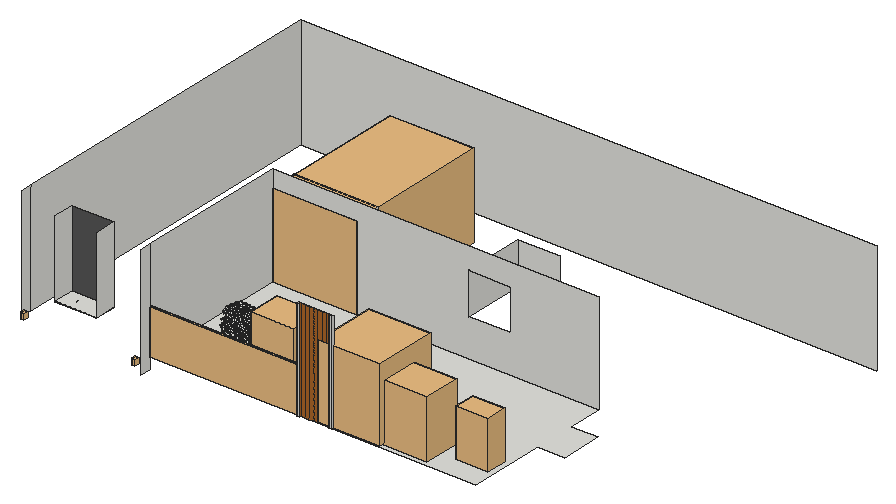
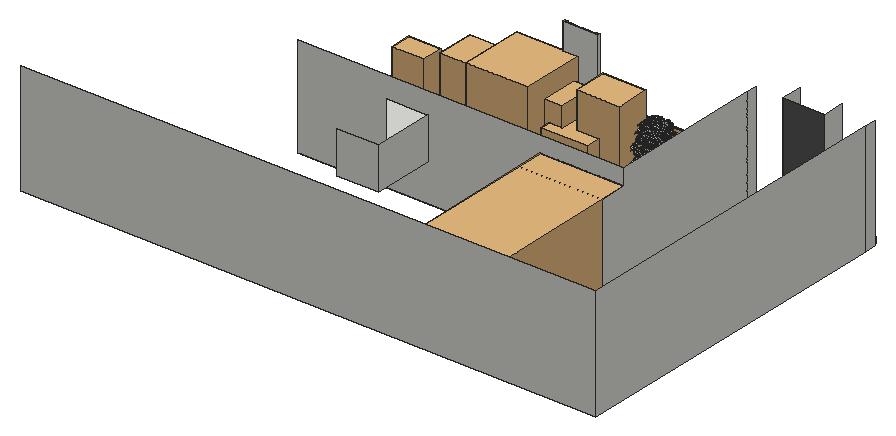
# SketchUp Ruby script. Lengths in inches.
U = 1.inch
M = Sketchup.active_model
def pt(a) = Geom::Point3d.new(a.map { |v| v * U })
def face(e, loops, mat)
  f = e.add_face(loops[0].map { |a| pt(a) })
  loops[1..].each { |l| e.add_face(l.map { |a| pt(a) }).erase! }
  f.material = f.back_material = mat if mat
  f
end
# faces: each face lists its corners as indices into pts; further lists are holes
def faces(e, pts, list, mat = nil) = list.each { |f| face(e, (f[0].is_a?(Array) ? f : [f]).map { |l| l.map { |i| pts[i] } }, mat) }
# xy, xz, yz: faces in a plane at the given z, y or x. An outline is a flat list of corners, or four numbers for a rectangle; further outlines are holes
def ring(l) = l.size == 4 ? [[l[0], l[1]], [l[2], l[1]], [l[2], l[3]], [l[0], l[3]]] : l.each_slice(2).to_a
def flat(e, list, mat, &to3) = list.each { |f| face(e, (f[0].is_a?(Array) ? f : [f]).map { |l| ring(l).map { |u, v| to3.(u, v) } }, mat) }
def xy(e, z, list, mat = nil) = flat(e, list, mat) { |x, y| [x, y, z] }
def xz(e, y, list, mat = nil) = flat(e, list, mat) { |x, z| [x, y, z] }
def yz(e, x, list, mat = nil) = flat(e, list, mat) { |y, z| [x, y, z] }
def lines(e, pts, list) = list.each { |a, b| e.add_line(pt(pts[a]), pt(pts[b])) }
# prism: a flat outline (further loops are holes) pulled along v
def prism(e, loops, v, mat = nil)
  f = face(e, loops, mat); d = Geom::Vector3d.new(v.map { |x| x * U })
  f.pushpull(f.normal.samedirection?(d) ? d.length : -d.length)
end
def box(e, o, s, mat = nil) = prism(e, [[o, [o[0] + s[0], o[1], o[2]], [o[0] + s[0], o[1] + s[1], o[2]], [o[0], o[1] + s[1], o[2]]]], [0, 0, s[2]], mat)
def at(x, y, z, deg = 0) = Geom::Transformation.translation(pt([x, y, z])) * Geom::Transformation.rotation(ORIGIN, Z_AXIS, deg.degrees)
def axes(o, x, y, z) = Geom::Transformation.new([*x, 0, *y, 0, *z, 0, *pt(o).to_a, 1])
def part(name) = M.definitions.add(name)
# library, detail: a bought-in or finely detailed component or shape, given as its bounding box
def library(name, o, s) = part(name).tap { |d| box(d.entities, o, s) }
def detail(e, o, s) = box(e.add_group.entities, o, s)
def put(e, d, t, mat = nil) = e.add_instance(d, t).tap { |i| i.material = mat if mat }
def group(e, t, mat = nil) = e.add_group.tap { |g| g.transformation = t; g.material = mat if mat }.entities
root = M.entities
M.materials.add("[Color M06]").color = [86, 86, 86]
M.materials.add("[Wood Bamboo]").color = [173, 103, 41]
c1 = library("Lamp Wall Outdoor 94-02",[-1.89,-4.65,-3.17],[3.78,4.65,6.35])
c2 = library("Omni Light",[-12,-12,-12],[24,24,24])
c3 = library("Group\#14",[0,0,0],[39.5,117.4375,51.17])
c4 = library("Glass Railings(black Handrails)",[-57.04,-132.55,0],[169.29,2.52,28.17])
c5 = library("Hanging Plant\#2",[-3.24,-1.74,-0.87],[34.15,22.4,50.98])
c6 = library("Yukka Plant GHD",[0,0,0],[46.13,35.26,75.51])
c7 = library("Philodendron Plant GHD",[-18.43,-10.97,-1.09],[51.75,39.48,62.43])
c8 = library("Plant Banana",[3.49,5.74,0],[38.27,39.55,56.51])
c9 = library("Potted indoor plant",[-35.72,-28.42,0],[66.31,67.39,78.4375])
c10 = part("leaflet")
p = [[2.87,10.24,0.32],[0.33,13.79,0],[-2.24,10.39,0.32],[-2.2,6.92,0.33],[0.45,0.11,0.33],[2.91,6.86,0.33]]
faces(c10.entities,p,[[0,1,2],[0,2,3,4,5]])
c11 = part("leaf group")
put(c11.entities,c10,axes([4.25,4.04,0.04],[0.8,0,0],[0,0.8,0],[0,0,0.8]))
put(c11.entities,c10,axes([4.5,3.78,0.04],[0.4,0.69282,-0.00011],[-0.69282,0.4,-0.00008],[-0.00001,0.00014,0.8]))
put(c11.entities,c10,axes([4.92,3.9375,0.04],[-0.56569,0.56569,-0.00025],[-0.56569,-0.56569,0.00001],[-0.00017,0.00019,0.8]))
put(c11.entities,c10,axes([4.87,4.38,0.04],[-0.69282,-0.4,-0.0002],[0.4,-0.69282,0.00017],[-0.00026,0.00005,0.8]))
put(c11.entities,c10,axes([4.42,4.45,0.04],[0.20706,-0.77274,-0.00003],[0.77274,0.20706,0.00016],[-0.00015,-0.00007,0.8]))
c12 = part("branch with leaves\#1")
put(c12.entities,c11,axes([2.86,31.23,35.15],[-0.02765,-0.79009,-0.61237],[0.48114,-0.54749,0.68465],[-0.8762,-0.27571,0.39528]))
put(c12.entities,c11,axes([12.72,29.5,24.05],[-0.41566,0.90952,0],[-0.44736,-0.20444,-0.87067],[-0.7919,-0.3619,0.49186]))
put(c12.entities,c11,axes([15.91,15.09,15.29],[-0.51919,0.82474,-0.22414],[0.78767,0.35997,-0.5],[-0.33169,-0.43615,-0.83652]))
put(c12.entities,c11,axes([23.4,16.37,17.31],[0.5,0.75,-0.43301],[0,0.5,0.86603],[0.86603,-0.43301,0.25]))
put(c12.entities,c11,axes([11.3125,8.27,23.62],[1.15,0,0],[0,0.575,0.99593],[0,-0.86603,0.5]))
c13 = part("leaflet\#1")
p = [[0.33,13.79,0],[2.87,10.24,0.32],[-2.24,10.39,0.32],[2.91,6.86,0.33],[0.45,0.11,0.33],[-2.2,6.92,0.33]]
faces(c13.entities,p,[[0,1,2],[2,1,3,4,5]])
c14 = part("leaf group\#1")
put(c14.entities,c13,axes([1.8,0.82,0.04],[-0.56569,0.56569,-0.00025],[-0.33941,-0.33941,0.00001],[-0.00017,0.00019,0.8]))
c15 = part("flower")
put(c15.entities,c14,axes([3.87,3.58,0.87],[0.08758,0.98061,-0.17532],[0.93721,-0.14075,-0.31909],[-0.33758,-0.13637,-0.93137]))
put(c15.entities,c14,axes([3.58,5.87,0.87],[0.98061,-0.08758,-0.17532],[-0.14075,-0.93721,-0.31909],[-0.13637,0.33758,-0.93137]))
put(c15.entities,c14,axes([5.87,6.16,0.87],[-0.08758,-0.98061,-0.17532],[-0.93721,0.14075,-0.31909],[0.33758,0.13637,-0.93137]))
put(c15.entities,c14,axes([6.16,3.87,0.87],[-0.98061,0.08758,-0.17532],[0.14075,0.93721,-0.31909],[0.13637,-0.33758,-0.93137]))
put(c15.entities,c14,axes([4.97,4.02,1.64],[-0.54077,0.62855,-0.55902],[0.78035,0.12673,-0.61237],[-0.31406,-0.76738,-0.55902]))
put(c15.entities,c14,axes([4.08,5.2,1.64],[0.81472,0.15405,-0.55902],[-0.28042,-0.73917,-0.61237],[-0.50754,0.65567,-0.55902]))
put(c15.entities,c14,axes([5.55,5.38,1.64],[-0.27395,-0.78259,-0.55902],[-0.49993,0.61243,-0.61237],[0.8216,0.11171,-0.55902]))
c16 = part("branch")
p = [[0.27,0.14,21.6],[1.15,1.36,21.6],[2.31,4.21,0],[0.54,1.79,0],[1.05,2.55,32.4],[1.34,2.95,32.4]]
faces(c16.entities,p,[[0,1,2,3],[4,5,1,0]])
c17 = part("branch with leaves")
put(c17.entities,c11,axes([29.28,4.46,29.75],[0.70711,0.61237,-0.35355],[-0.27393,0.69819,0.66144],[0.65189,-0.37086,0.66144]))
put(c17.entities,c11,axes([2.86,31.23,35.15],[-0.02765,-0.79009,-0.61237],[0.48114,-0.54749,0.68465],[-0.8762,-0.27571,0.39528]))
put(c17.entities,c16,axes([15.22,43.9,5.2],[1,0,0],[0,0.5,0.86603],[0,-1.03923,0.6]))
put(c17.entities,c11,axes([12.72,29.5,24.05],[-0.41566,0.90952,0],[-0.44736,-0.20444,-0.87067],[-0.7919,-0.3619,0.49186]))
put(c17.entities,c11,axes([15.91,15.09,15.29],[-0.51919,0.82474,-0.22414],[0.78767,0.35997,-0.5],[-0.33169,-0.43615,-0.83652]))
put(c17.entities,c11,axes([31.61,42.03,14.23],[-0.02765,-0.79009,-0.61237],[0.47126,0.52995,-0.70503],[0.88156,-0.30808,0.35768]))
put(c17.entities,c11,axes([23.4,16.37,17.31],[0.5,0.75,-0.43301],[0,0.5,0.86603],[0.86603,-0.43301,0.25]))
put(c17.entities,c11,axes([12.04,8.6,24.1875],[1,0,0],[0,0.5,0.86603],[0,-0.86603,0.5]))
c18 = part("trunk")
p = [[2.07,0,0],[2.91,2.57,208.4],[2.76,2.68,208.4],[0.57,1.09,0],[3.93,0,0],[3.09,2.57,208.4],
  [5.43,1.09,0],[3.24,2.68,208.4],[2.7,2.85,208.4],[0,2.85,0],[6,2.85,0],[3.3,2.85,208.4],
  [2.76,3.03,208.4],[0.57,4.62,0],[5.43,4.62,0],[3.24,3.03,208.4],[2.91,3.14,208.4],[2.07,5.71,0],
  [3.93,5.71,0],[3.09,3.14,208.4]]
faces(c18.entities,p,[[0,1,2,3],[4,5,1,0],[6,7,5,4],[3,2,8,9],[6,10,11,7],[8,12,13,9],[11,10,14,15],[13,12,16,17],
  [18,19,15,14],[17,16,19,18]])
c19 = part("Flowering tree")
put(c19.entities,c12,axes([8.5625,69.79,58.85],[-1.14545,-0.10223,0],[0.09875,-1.10642,-0.25882],[0.02646,-0.29646,0.96593]))
put(c19.entities,c15,axes([18.03,-59.9,126.47],[-1.06473,0.02061,0.37747],[-0.32263,-0.80708,-0.6548],[0.29115,-0.81896,0.6548]))
put(c19.entities,c15,axes([24.99,-51.52,163.52],[0.99593,0.2875,-0.43301],[0,0.99593,0.5],[0.575,-0.49796,0.75]))
put(c19.entities,c15,axes([9.15,43.86,180.9375],[-0.776,0.32151,0.68301],[0.59221,-0.55726,0.70711],[0.60796,0.9532,0.18301]))
put(c19.entities,c15,axes([-19.44,51.82,88.4375],[-0.978,0.2192,-0.49033],[-0.25151,-1.12216,0],[-0.55023,0.12332,0.87153]))
put(c19.entities,c12,axes([79.24,-48.01,132.64],[0.21275,1.12031,-0.12941],[-1.10684,0.17595,-0.22414],[-0.22834,0.19092,0.96593]))
put(c19.entities,c12,axes([64.36,-6.43,165.85],[-0.10223,1.14545,0],[-1.10642,-0.09875,-0.25882],[-0.29646,-0.02646,0.96593]))
put(c19.entities,c12,axes([52.57,39.62,163.85],[-0.88224,0.73767,0],[-0.71253,-0.85218,-0.25882],[-0.19092,-0.22834,0.96593]))
put(c19.entities,c12,axes([-64.4,-29.26,175.85],[0.88224,-0.73767,0],[0.71253,0.85218,-0.25882],[0.19092,0.22834,0.96593]))
put(c19.entities,c12,axes([40.35,-16.55,200.81],[-0.14358,1.14093,0.01256],[-0.77283,-0.08933,-0.72016],[-0.83795,-0.11311,0.69546]))
put(c19.entities,c12,axes([7.875,84.56,112.85],[-1.14773,-0.07221,0],[0.06975,-1.10862,-0.25882],[0.01869,-0.29705,0.96593]))
put(c19.entities,c12,axes([-66.42,6.43,163.85],[0.10223,-1.14545,0],[1.10642,0.09875,-0.25882],[0.29646,0.02646,0.96593]))
put(c19.entities,c12,axes([-6.02,-66.82,162.85],[1.14545,0.10223,0],[-0.09875,1.10642,-0.25882],[-0.02646,0.29646,0.96593]))
put(c19.entities,c12,axes([65.22,55.72,70.85],[-0.88224,0.73767,0],[-0.71253,-0.85218,-0.25882],[-0.19092,-0.22834,0.96593]))
put(c19.entities,c12,axes([-6.02,-85.22,100.85],[1.14545,0.10223,0],[-0.09875,1.10642,-0.25882],[-0.02646,0.29646,0.96593]))
put(c19.entities,c12,axes([-64.4,-55.71,70.85],[0.88224,-0.73767,0],[0.71253,0.85218,-0.25882],[0.19092,0.22834,0.96593]))
put(c19.entities,c12,axes([-46.27,-12.7,180.74],[-0.29529,-0.0373,-0.96593],[1.10206,0.13922,-0.25882],[0.14413,-1.14093,0]))
put(c19.entities,c12,axes([56.125,-64.81,70.85],[0.73767,0.88224,0],[-0.85218,0.71253,-0.25882],[-0.22834,0.19092,0.96593]))
put(c19.entities,c12,axes([-55.31,64.8125,78.85],[-0.73767,-0.88224,0],[0.85218,-0.71253,-0.25882],[0.22834,-0.19092,0.96593]))
put(c19.entities,c12,axes([-84.82,6.43,92.85],[0.10223,-1.14545,0],[1.10642,0.09875,-0.25882],[0.29646,0.02646,0.96593]))
put(c19.entities,c17,axes([56.87,3.27,57.34],[-0.44564,1.06014,0],[-1.06014,-0.44564,0],[0,0,1]))
put(c19.entities,c15,axes([-46.02,24.68,176.39],[-0.60389,-0.88348,0.36612],[0.59197,0.06424,0.85552],[-0.77935,0.73337,0.36612]))
put(c19.entities,c17,axes([-18.99,-54,51.28],[1.15,0,0],[0,1.15,0],[0,0,1]))
put(c19.entities,c15,axes([-14.26,69.05,133.89],[-0.21654,-1.04563,0.37124],[1.09634,-0.09014,0.29155],[-0.27139,0.47014,0.88158]))
put(c19.entities,c12,axes([7.875,59.26,173.85],[-1.14773,-0.07221,0],[0.06975,-1.10862,-0.25882],[0.01869,-0.29705,0.96593]))
put(c19.entities,c15,axes([-39.65,-46.59,156.55],[0.81317,-0.40659,0.61237],[0,0.99593,0.5],[-0.81317,-0.40659,0.61237]))
put(c19.entities,c12,axes([68.45,-14.73,133.12],[0.31285,1.10009,0.10445],[-1.0665,0.33304,-0.23681],[-0.29529,-0.0373,0.96593]))
put(c19.entities,c17,axes([-54.71,-13.99,125.23],[0.64805,-0.95001,0],[0.91764,0.62597,-0.25882],[0.24588,0.16773,0.96593]))
put(c19.entities,c15,axes([-59.37,-17.76,103.29],[0.82621,-0.65851,-0.39489],[0.59197,0.06424,0.85552],[-0.538,-0.9406,0.33489]))
put(c19.entities,c17,axes([-55.12,-14.55,89.35],[0.64805,-0.95001,0],[0.91764,0.62597,-0.25882],[0.24588,0.16773,0.96593]))
put(c19.entities,c15,axes([48.53,-28.74,71.58],[0.35234,0.10813,0.94725],[-0.36862,-1.06582,0.19567],[1.03076,-0.41812,-0.25382]))
put(c19.entities,c12,axes([-12.83,63.67,197.61],[0.0612,-1.14229,0.10265],[-1.10726,-0.09004,-0.2585],[0.30453,-0.09784,-0.96054]))
put(c19.entities,c12,axes([-64.4,-55.71,112.85],[0.88224,-0.73767,0],[0.71253,0.85218,-0.25882],[0.19092,0.22834,0.96593]))
put(c19.entities,c12,axes([65.22,55.72,114.85],[-0.88224,0.73767,0],[-0.71253,-0.85218,-0.25882],[-0.19092,-0.22834,0.96593]))
put(c19.entities,c15,axes([63.34,2.95,120.74],[0.8666,0.37799,-0.5693],[-0.45977,1.05409,0],[0.6001,0.26175,0.82213]))
put(c19.entities,c12,axes([85.63,-6.43,94.85],[-0.10223,1.14545,0],[-1.10642,-0.09875,-0.25882],[-0.29646,-0.02646,0.96593]))
put(c19.entities,c17,axes([31.42,47.13,103.94],[-1.11535,0.28016,0],[-0.27473,-1.09373,-0.19595],[-0.0549,-0.21855,0.98061]))
put(c19.entities,c18,axes([-3.39,-3.28,43.76],[1.15,0,0],[0,1.15,0],[0,0,0.79]))
put(c19.entities,c17,axes([34.9,-44.92,95.18],[0.62465,0.96556,0],[-0.93266,0.60337,-0.25882],[-0.24991,0.16167,0.96593]))
put(c19.entities,c17,axes([32.7,-43.8,134.99],[0.62465,0.96556,0],[-0.88615,0.57328,-0.39715],[-0.38347,0.24808,0.91775]))
put(c19.entities,c12,axes([-51.54,49.67,143.57],[0.26379,-0.52212,-0.86096],[0.65423,-0.75347,0.49708],[-0.90824,-0.69439,0.108]))
put(c19.entities,c17,axes([31.48,46.68,140.85],[-1.11535,0.28016,0],[-0.27061,-1.07735,-0.25882],[-0.07251,-0.28867,0.96593]))
put(c19.entities,c12,axes([8.75,19.55,179.21],[-0.27543,0.79346,0.68307],[-1.10726,-0.09004,-0.2585],[-0.14361,-0.82754,0.68307]))
c20 = part("Plant GHD")
put(c20.entities,c19,axes([21.36,20.42,-5.32],[0.2847,0,0],[0,0.2847,0],[0,0,0.33025]))
g1 = group(c20.entities,at(14.85,13.9,0))
detail(g1,[0,0,0],[13.04,13.04,11.8])
c21 = library("Group\#719",[-5.55,-6.67,0],[49.65,49.64,35.75])
c22 = part("Plants indoor GHD")
put(c22.entities,c5,at(254.34,21.02,0))
put(c22.entities,c6,at(45.23,2.59,0))
put(c22.entities,c7,at(201.7,11.53,0))
put(c22.entities,c8,at(99.46,-3.08,1.17))
put(c22.entities,c9,at(158.24,24.68,0))
put(c22.entities,c20,at(0,0,0))
put(c22.entities,c21,at(72.51,10.66,1.17))
xy(root,124.51,[[782.66,915.1875,785.84,916.1875],[817.03,915.1875,820.03,916.1875],[624.25,916.1875,782.66,916.1875,782.66,917.0625,820.03,917.0625,820.03,916.1875,973.0625,916.1875,973.0625,998.1875,1001.875,998.1875,1001.875,1042.875,973.0625,1042.875,973.0625,1080.1875,714.02,1080.1875,714.02,1109,624.25,1109],[782.66,916.1875,820.03,917.0625]])
xy(root,158.17,[[541.1875,893.4375,586.375,916.1875]])
xy(root,158.97,[[541.1875,893.4375,586.375,916.1875]])
xz(root,893.4375,[[541.1875,158.17,586.375,158.97]])
xz(root,915.1875,[[782.66,124.51,785.84,232.51],[817.03,124.51,820.03,232.51]])
xz(root,916.1875,[[541.1875,158.97,586.375,240.28]],"[Color M06]")
xz(root,916.1875,[[785.84,124.51,790.3,232.51],[790.3,124.51,794.75,232.51],[794.75,124.51,799.21,232.51],[799.21,124.51,803.67,232.51],[803.67,124.51,808.12,232.51],
  [808.12,124.51,812.58,232.51],[812.58,124.51,817.03,232.51]],"[Wood Bamboo]")
xz(root,917.0625,[[782.66,124.51,820.03,232.51]])
xz(root,1080.1875,[[[714.02,124.51,973.0625,124.51,973.0625,232.51,624.25,232.51,624.25,214.57,714.02,214.57],[834.07,164.6,878.82,209.35]]])
xz(root,1109,[[624.25,124.51,714.02,214.57]])
xz(root,1146.3125,[[834.07,164.6,878.82,209.35]])
xz(root,1276.1875,[[497.625,124.51,1112.75,244.51]])
yz(root,497.625,[[904.1875,124.51,916.1875,244.51],[916.1875,124.51,1276.1875,244.51]])
yz(root,541.1875,[[893.4375,158.97,916.1875,240.28]])
yz(root,586.375,[[893.4375,158.97,916.1875,240.28]])
yz(root,624.25,[[904.1875,112.51,916.1875,232.51],[916.1875,124.51,1109,124.51,1109,214.57,1080.1875,214.57,1080.1875,232.51,916.1875,232.51]])
yz(root,714.02,[[1080.1875,124.51,1109,214.57]])
yz(root,782.66,[[915.1875,124.51,917.0625,232.51]])
yz(root,785.84,[[915.1875,124.51,916.1875,232.51]],"[Wood Bamboo]")
yz(root,817.03,[[915.1875,124.51,916.1875,232.51]],"[Wood Bamboo]")
yz(root,820.03,[[915.1875,124.51,917.0625,232.51]])
yz(root,834.07,[[1080.1875,164.6,1146.3125,209.35]])
put(root,c1,at(501.36,904.1875,127.53))
put(root,c2,axes([557.7,904.27,156.48],[0.14094,0,0],[0,0.14094,0],[0,0,0.14094]))
put(root,c1,at(620.45,904.1875,125.27))
put(root,c3,axes([624.35,1080.1875,124.51],[2.27,0,0],[0,1.34,0],[0,0,1.75999]))
put(root,c4,axes([677.63,1048.73,124.51],[0.9357,0,0],[0,1,0],[0,0,1.70393]))
put(root,c22,at(681.97,919.92,125.62))
